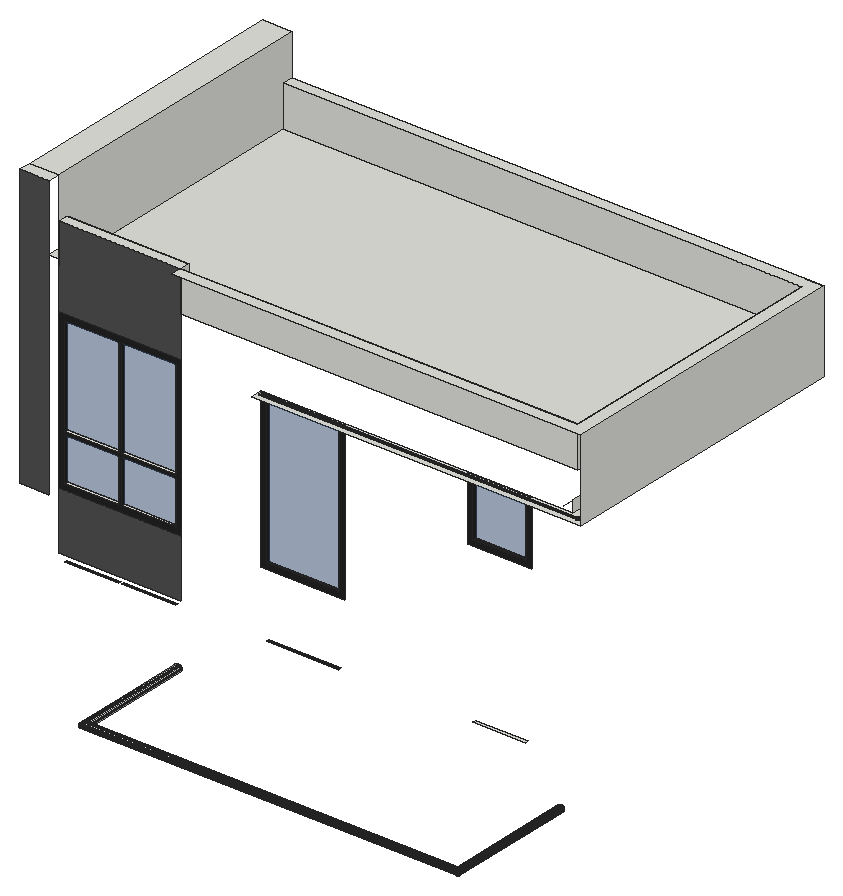
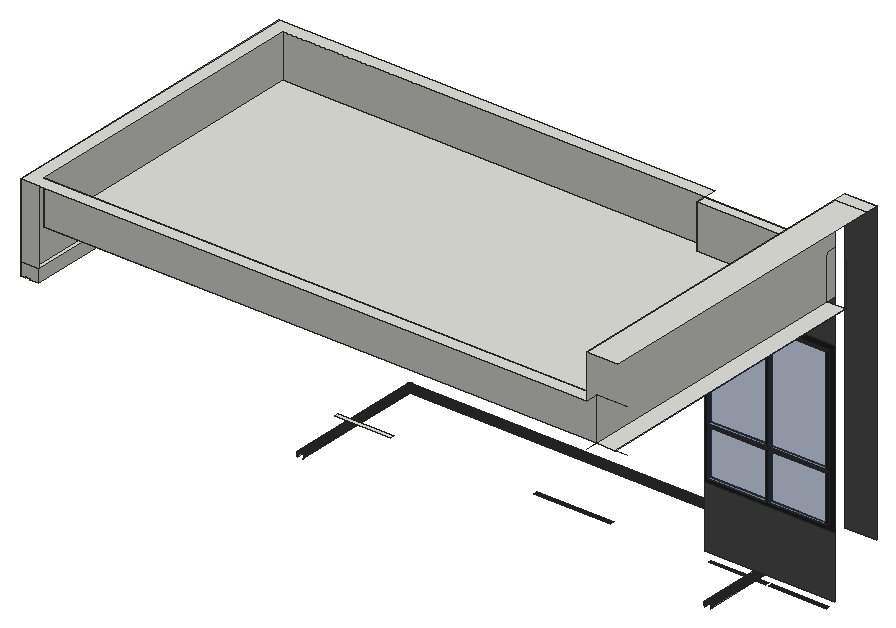
# SketchUp Ruby script. Lengths in inches.
U = 1.inch
M = Sketchup.active_model
def pt(a) = Geom::Point3d.new(a.map { |v| v * U })
def face(e, loops, mat)
  f = e.add_face(loops[0].map { |a| pt(a) })
  loops[1..].each { |l| e.add_face(l.map { |a| pt(a) }).erase! }
  f.material = f.back_material = mat if mat
  f
end
# faces: each face lists its corners as indices into pts; further lists are holes
def faces(e, pts, list, mat = nil) = list.each { |f| face(e, (f[0].is_a?(Array) ? f : [f]).map { |l| l.map { |i| pts[i] } }, mat) }
# xy, xz, yz: faces in a plane at the given z, y or x. An outline is a flat list of corners, or four numbers for a rectangle; further outlines are holes
def ring(l) = l.size == 4 ? [[l[0], l[1]], [l[2], l[1]], [l[2], l[3]], [l[0], l[3]]] : l.each_slice(2).to_a
def flat(e, list, mat, &to3) = list.each { |f| face(e, (f[0].is_a?(Array) ? f : [f]).map { |l| ring(l).map { |u, v| to3.(u, v) } }, mat) }
def xy(e, z, list, mat = nil) = flat(e, list, mat) { |x, y| [x, y, z] }
def xz(e, y, list, mat = nil) = flat(e, list, mat) { |x, z| [x, y, z] }
def yz(e, x, list, mat = nil) = flat(e, list, mat) { |y, z| [x, y, z] }
def lines(e, pts, list) = list.each { |a, b| e.add_line(pt(pts[a]), pt(pts[b])) }
# prism: a flat outline (further loops are holes) pulled along v
def prism(e, loops, v, mat = nil)
  f = face(e, loops, mat); d = Geom::Vector3d.new(v.map { |x| x * U })
  f.pushpull(f.normal.samedirection?(d) ? d.length : -d.length)
end
def box(e, o, s, mat = nil) = prism(e, [[o, [o[0] + s[0], o[1], o[2]], [o[0] + s[0], o[1] + s[1], o[2]], [o[0], o[1] + s[1], o[2]]]], [0, 0, s[2]], mat)
def at(x, y, z, deg = 0) = Geom::Transformation.translation(pt([x, y, z])) * Geom::Transformation.rotation(ORIGIN, Z_AXIS, deg.degrees)
def axes(o, x, y, z) = Geom::Transformation.new([*x, 0, *y, 0, *z, 0, *pt(o).to_a, 1])
def part(name) = M.definitions.add(name)
# library, detail: a bought-in or finely detailed component or shape, given as its bounding box
def library(name, o, s) = part(name).tap { |d| box(d.entities, o, s) }
def detail(e, o, s) = box(e.add_group.entities, o, s)
def put(e, d, t, mat = nil) = e.add_instance(d, t).tap { |i| i.material = mat if mat }
def group(e, t, mat = nil) = e.add_group.tap { |g| g.transformation = t; g.material = mat if mat }.entities
root = M.entities
M.materials.add("[0033_NavajoWhite]").color = [226, 197, 153]
M.materials.add("[0136_Charcoal]").color = [35, 35, 35]
M.materials.add("[Cladding Siding White]2").color = [81, 81, 81]
M.materials.add("[Translucent Glass Blue]").color = [52, 78, 124]
M.materials["[Translucent Glass Blue]"].alpha = 0.5
xy(root,1728,[[912,288,1020,294]])
xy(root,1728,[[72,288,183,294],[189,288,300,294],[487.9375,288,636,294]],"[0136_Charcoal]")
xy(root,1872,[[72,288,183,295],[189,288,300,295]])
xy(root,1872,[[487.9375,288,636,294]],"[0136_Charcoal]")
xy(root,1962,[[72,288,183,295],[189,288,300,295]],"[0136_Charcoal]")
xy(root,1968,[[72,288,183,295],[189,288,300,295]])
xy(root,2064,[[912,288,1020,294]],"[0136_Charcoal]")
xy(root,2172,[[72,288,183,295],[189,288,300,295],[487.9375,288,636,294],[912,288,1020,294]],"[0136_Charcoal]")
xy(root,2184,[[475.9375,264,475.9375,288,1116,288,1116,888,1134,888,1134,285.66,1133.95,284.93,1133.81,284.21,1133.57,283.51,1133.25,282.85,1132.84,282.24,1132.35,281.68,1131.8,281.2,1131.1875,280.79,1130.53,280.46,1129.83,280.23,1129.11,280.08,1128.37,280.03,481.92,280.03,481.92,275.66,1132,275.66,1133.2,275.74,1134.375,275.97,1135.51,276.36,1136.58,276.89,1137.58,277.55,1138.48,278.35,1139.27,279.25,1139.94,280.25,1140.47,281.32,1140.86,282.46,1141.09,283.63,1141.17,284.83,1141.17,888,1152,888,1152,264]])
xy(root,2186,[[481.92,275.66,481.92,280.03,1128.37,280.03,1129.11,280.08,1129.83,280.23,1130.53,280.46,1131.1875,280.79,1131.8,281.2,1132.35,281.68,1132.84,282.24,1133.25,282.85,1133.57,283.51,1133.81,284.21,1133.95,284.93,1134,285.66,1134,888,1141.17,888,1141.17,284.83,1141.09,283.63,1140.86,282.46,1140.47,281.32,1139.94,280.25,1139.27,279.25,1138.48,278.35,1137.58,277.55,1136.58,276.89,1135.51,276.36,1134.375,275.97,1133.2,275.74,1132,275.66]],"[0033_NavajoWhite]")
xy(root,2268,[[312,288,1126,288,1126,864,60,864,60,308,312,308],[23.25,308,24,864],[24,308,60,864]])
xy(root,2352,[[312,264,1152,264,1152,888,60,888,60,864,1126,864,1126,288,312,288],[60,288,312,308]])
xy(root,2436,[[0,264,60,288],[0,288,60,888]])
xz(root,264,[[0,1858.15,60,2436]],"[Cladding Siding White]2")
xz(root,275.66,[[481.92,2184,1132,2186]])
xz(root,280.03,[[481.92,2184,1128.37,2186]])
xz(root,288,[[312,2268,1126,2352]])
xz(root,288,[[[60,1860,312,2184],[189,1968,300,2172],[72,1968,183,2172],[72,1872,183,1962],[189,1872,300,1962]],[[475.9375,1860,648,2184],[487.9375,1872,636,2172]],[[900,2052,1032,2184],[912,2064,1020,2172]]],"[0136_Charcoal]")
xz(root,288,[[60,1740,312,1860],[60,2184,312,2352]],"[Cladding Siding White]2")
xz(root,294,[[487.9375,1872,636,2172],[912,2064,1020,2172]],"[Translucent Glass Blue]")
xz(root,295,[[72,1872,183,1962],[189,1872,300,1962],[72,1968,183,2172],[189,1968,300,2172]],"[Translucent Glass Blue]")
xz(root,308,[[60,2268,312,2352]])
xz(root,864,[[60,2268,1126,2352]])
xz(root,888,[[1116,2184,1116,2208,1152,2208,1152,2184,1141.17,2184,1141.17,2186,1134,2186,1134,2184],[1116,2208,1152,2352]])
yz(root,60,[[288,2268,308,2352],[308,2268,864,2268,864,2352,888,2352,888,2436,288,2436,288,2352,308,2352]])
yz(root,72,[[288,1872,295,1962],[288,1968,295,2172]],"[0136_Charcoal]")
yz(root,183,[[288,1872,295,1962],[288,1968,295,2172]],"[0136_Charcoal]")
yz(root,189,[[288,1872,295,1962],[288,1968,295,2172]],"[0136_Charcoal]")
yz(root,300,[[288,1872,295,1962],[288,1968,295,2172]],"[0136_Charcoal]")
yz(root,312,[[288,2268,308,2352]])
yz(root,481.92,[[275.66,2184,280.03,2186]])
yz(root,487.9375,[[288,1872,294,2172]],"[0136_Charcoal]")
yz(root,636,[[288,1872,294,2172]],"[0136_Charcoal]")
yz(root,912,[[288,2064,294,2172]],"[0136_Charcoal]")
yz(root,1020,[[288,2064,294,2172]],"[0136_Charcoal]")
yz(root,1116,[[288,2184,888,2208]])
yz(root,1126,[[288,2268,864,2352]])
yz(root,1134,[[285.66,2184,888,2186]])
yz(root,1141.17,[[284.83,2184,888,2186]])
yz(root,1152,[[264,2184,888,2352]])
p = [[319.57,264,1627.89],[320.03,264,1627.32],[320.03,18.8,1627.32],[319.57,18.34,1627.89],[1097.35,18.8,1627.32],[1097.81,18.34,1627.89],
  [1097.35,288,1627.32],[1097.81,288,1627.89],[330.43,264,1627.32],[330.9,264,1627.89],[330.9,29.66,1627.89],[330.43,29.2,1627.32],
  [1086.48,29.66,1627.89],[1086.94,29.2,1627.32],[1086.48,288,1627.89],[1086.94,288,1627.32],[319.17,264,1628.5],[319.17,17.9375,1628.5],
  [1098.21,17.9375,1628.5],[1098.21,288,1628.5],[331.29,264,1628.5],[331.29,30.0625,1628.5],[1086.08,30.0625,1628.5],[1086.08,288,1628.5],
  [318.84,264,1629.15],[318.84,17.61,1629.15],[1098.54,17.61,1629.15],[1098.54,288,1629.15],[331.63,264,1629.15],[331.63,30.39,1629.15],
  [1085.75,30.39,1629.15],[1085.75,288,1629.15],[318.58,264,1629.84],[318.58,17.34,1629.84],[1098.8,17.34,1629.84],[1098.8,288,1629.84],
  [331.89,264,1629.84],[331.89,30.66,1629.84],[1085.49,30.66,1629.84],[1085.49,288,1629.84],[318.39,264,1630.54],[318.39,17.15,1630.54],
  [1098.99,17.15,1630.54],[1098.99,288,1630.54],[332.08,264,1630.54],[332.08,30.85,1630.54],[1085.3,30.85,1630.54],[1085.3,288,1630.54],
  [318.27,264,1631.27],[318.27,17.04,1631.27],[1099.11,17.04,1631.27],[1099.11,288,1631.27],[332.19,264,1631.27],[332.19,30.96,1631.27],
  [1085.18,30.96,1631.27],[1085.18,288,1631.27],[318.23,264,1632],[318.23,17,1632],[1099.15,17,1632],[1099.15,288,1632],
  [332.23,264,1632],[332.23,31,1632],[1085.15,31,1632],[1085.15,288,1632],[318.27,264,1632.73],[318.27,17.04,1632.73],
  [1099.11,17.04,1632.73],[1099.11,288,1632.73],[332.19,264,1632.73],[332.19,30.96,1632.73],[1085.18,30.96,1632.73],[1085.18,288,1632.73],
  [318.39,264,1633.46],[318.39,17.15,1633.46],[1098.99,17.15,1633.46],[1098.99,288,1633.46],[332.08,264,1633.46],[332.08,30.85,1633.46],
  [1085.3,30.85,1633.46],[1085.3,288,1633.46],[318.58,264,1634.16],[318.58,17.34,1634.16],[1098.8,17.34,1634.16],[1098.8,288,1634.16],
  [331.89,264,1634.16],[331.89,30.66,1634.16],[1085.49,30.66,1634.16],[1085.49,288,1634.16],[318.84,264,1634.85],[318.84,17.61,1634.85],
  [1098.54,17.61,1634.85],[1098.54,288,1634.85],[331.63,264,1634.85],[331.63,30.39,1634.85],[1085.75,30.39,1634.85],[1085.75,288,1634.85],
  [319.17,264,1635.5],[319.17,17.9375,1635.5],[1098.21,17.9375,1635.5],[1098.21,288,1635.5],[331.29,264,1635.5],[331.29,30.0625,1635.5],
  [1086.08,30.0625,1635.5],[1086.08,288,1635.5],[319.57,264,1636.11],[319.57,18.34,1636.11],[1097.81,18.34,1636.11],[1097.81,288,1636.11],
  [330.9,264,1636.11],[330.9,29.66,1636.11],[1086.48,29.66,1636.11],[1086.48,288,1636.11],[320.03,264,1636.68],[320.03,18.8,1636.68],
  [1097.35,18.8,1636.68],[1097.35,288,1636.68],[330.43,264,1636.68],[330.43,29.2,1636.68],[1086.94,29.2,1636.68],[1086.94,288,1636.68],
  [320.55,264,1637.2],[320.55,19.32,1637.2],[1096.83,19.32,1637.2],[1096.83,288,1637.2],[329.92,264,1637.2],[329.92,28.68,1637.2],
  [1087.46,28.68,1637.2],[1087.46,288,1637.2],[321.12,264,1637.66],[321.12,19.89,1637.66],[1096.26,19.89,1637.66],[1096.26,288,1637.66],
  [329.35,264,1637.66],[329.35,28.11,1637.66],[1088.03,28.11,1637.66],[1088.03,288,1637.66],[321.73,264,1638.0625],[321.73,20.5,1638.0625],
  [1095.65,20.5,1638.0625],[1095.65,288,1638.0625],[328.73,264,1638.0625],[328.73,27.5,1638.0625],[1088.65,27.5,1638.0625],[1088.65,288,1638.0625],
  [322.39,264,1638.39],[322.39,21.15,1638.39],[1094.99,21.15,1638.39],[1094.99,288,1638.39],[328.08,264,1638.39],[328.08,26.85,1638.39],
  [1089.3,26.85,1638.39],[1089.3,288,1638.39],[323.07,264,1638.66],[323.07,21.84,1638.66],[1094.31,21.84,1638.66],[1094.31,288,1638.66],
  [327.4,264,1638.66],[327.4,26.16,1638.66],[1089.98,26.16,1638.66],[1089.98,288,1638.66],[323.78,264,1638.85],[323.78,22.54,1638.85],
  [1093.6,22.54,1638.85],[1093.6,288,1638.85],[326.6875,264,1638.85],[326.6875,25.46,1638.85],[1090.69,25.46,1638.85],[1090.69,288,1638.85],
  [324.5,264,1638.96],[324.5,23.27,1638.96],[1092.88,23.27,1638.96],[1092.88,288,1638.96],[325.96,264,1638.96],[325.96,24.73,1638.96],
  [1091.41,24.73,1638.96],[1091.41,288,1638.96],[325.23,264,1639],[325.23,24,1639],[1092.15,24,1639],[1092.15,288,1639],
  [1133.2,275.74,2184],[1132,275.66,2184],[1132,275.66,2186],[1133.2,275.74,2186],[1134.375,275.97,2184],[1134.375,275.97,2186],
  [1135.51,276.36,2184],[1135.51,276.36,2186],[1136.58,276.89,2184],[1136.58,276.89,2186],[1137.58,277.55,2184],[1137.58,277.55,2186],
  [1138.48,278.35,2184],[1138.48,278.35,2186],[1139.27,279.25,2184],[1139.27,279.25,2186],[1139.94,280.25,2184],[1139.94,280.25,2186],
  [1128.37,280.03,2184],[1129.11,280.08,2184],[1129.11,280.08,2186],[1128.37,280.03,2186],[1129.83,280.23,2184],[1129.83,280.23,2186],
  [1130.53,280.46,2184],[1130.53,280.46,2186],[1140.47,281.32,2184],[1140.47,281.32,2186],[1131.1875,280.79,2184],[1131.1875,280.79,2186],
  [1131.8,281.2,2184],[1131.8,281.2,2186],[1132.35,281.68,2184],[1132.35,281.68,2186],[1140.86,282.46,2184],[1140.86,282.46,2186],
  [1132.84,282.24,2184],[1132.84,282.24,2186],[1133.25,282.85,2184],[1133.25,282.85,2186],[1141.09,283.63,2184],[1141.09,283.63,2186],
  [1133.57,283.51,2184],[1133.57,283.51,2186],[1133.81,284.21,2184],[1133.81,284.21,2186],[1141.17,284.83,2184],[1141.17,284.83,2186],
  [1133.95,284.93,2184],[1133.95,284.93,2186],[1134,285.66,2184],[1134,285.66,2186],[1116,288,2208],[1116,264,2208],
  [0,864,2352],[60,864,2352],[60,864,2268],[60,888,2268],[23.25,308,2268],[23.25,308,2352],
  [23.25,864,2268],[0,864,2268]]
faces(root,p,[[0,1,2,3],[3,2,4,5],[5,4,6,7],[8,9,10,11],[11,10,12,13],[13,12,14,15],[16,0,3,17],[17,3,5,18],
  [18,5,7,19],[9,20,21,10],[10,21,22,12],[12,22,23,14],[24,16,17,25],[25,17,18,26],[26,18,19,27],[20,28,29,21],
  [21,29,30,22],[22,30,31,23],[32,24,25,33],[33,25,26,34],[34,26,27,35],[28,36,37,29],[29,37,38,30],[30,38,39,31],
  [40,32,33,41],[41,33,34,42],[42,34,35,43],[36,44,45,37],[37,45,46,38],[38,46,47,39],[48,40,41,49],[49,41,42,50],
  [50,42,43,51],[44,52,53,45],[45,53,54,46],[46,54,55,47],[56,48,49,57],[57,49,50,58],[58,50,51,59],[52,60,61,53],
  [53,61,62,54],[54,62,63,55],[64,56,57,65],[65,57,58,66],[66,58,59,67],[60,68,69,61],[61,69,70,62],[62,70,71,63],
  [72,64,65,73],[73,65,66,74],[74,66,67,75],[68,76,77,69],[69,77,78,70],[70,78,79,71],[80,72,73,81],[81,73,74,82],
  [82,74,75,83],[76,84,85,77],[77,85,86,78],[78,86,87,79],[88,80,81,89],[89,81,82,90],[90,82,83,91],[84,92,93,85],
  [85,93,94,86],[86,94,95,87],[96,88,89,97],[97,89,90,98],[98,90,91,99],[92,100,101,93],[93,101,102,94],[94,102,103,95],
  [104,96,97,105],[105,97,98,106],[106,98,99,107],[100,108,109,101],[101,109,110,102],[102,110,111,103],[112,104,105,113],[113,105,106,114],
  [114,106,107,115],[108,116,117,109],[109,117,118,110],[110,118,119,111],[120,112,113,121],[121,113,114,122],[122,114,115,123],[116,124,125,117],
  [117,125,126,118],[118,126,127,119],[128,120,121,129],[129,121,122,130],[130,122,123,131],[124,132,133,125],[125,133,134,126],[126,134,135,127],
  [136,128,129,137],[137,129,130,138],[138,130,131,139],[132,140,141,133],[133,141,142,134],[134,142,143,135],[144,136,137,145],[145,137,138,146],
  [146,138,139,147],[140,148,149,141],[141,149,150,142],[142,150,151,143],[152,144,145,153],[153,145,146,154],[154,146,147,155],[148,156,157,149],
  [149,157,158,150],[150,158,159,151],[160,152,153,161],[161,153,154,162],[162,154,155,163],[156,164,165,157],[157,165,166,158],[158,166,167,159],
  [168,160,161,169],[169,161,162,170],[170,162,163,171],[164,172,173,165],[165,173,174,166],[166,174,175,167],[176,168,169,177],[177,169,170,178],
  [178,170,171,179],[172,176,177,173],[173,177,178,174],[174,178,179,175],[180,181,182,183],[184,180,183,185],[186,184,185,187],[188,186,187,189],
  [190,188,189,191],[192,190,191,193],[194,192,193,195],[196,194,195,197],[198,199,200,201],[199,202,203,200],[202,204,205,203],[206,196,197,207],
  [204,208,209,205],[208,210,211,209],[210,212,213,211],[214,206,207,215],[212,216,217,213],[216,218,219,217],[220,214,215,221],[218,222,223,219],
  [222,224,225,223],[226,220,221,227],[224,228,229,225],[228,230,231,229]])
lines(root,p,[[232,233],[234,235],[236,237],[238,239],[240,241]])
